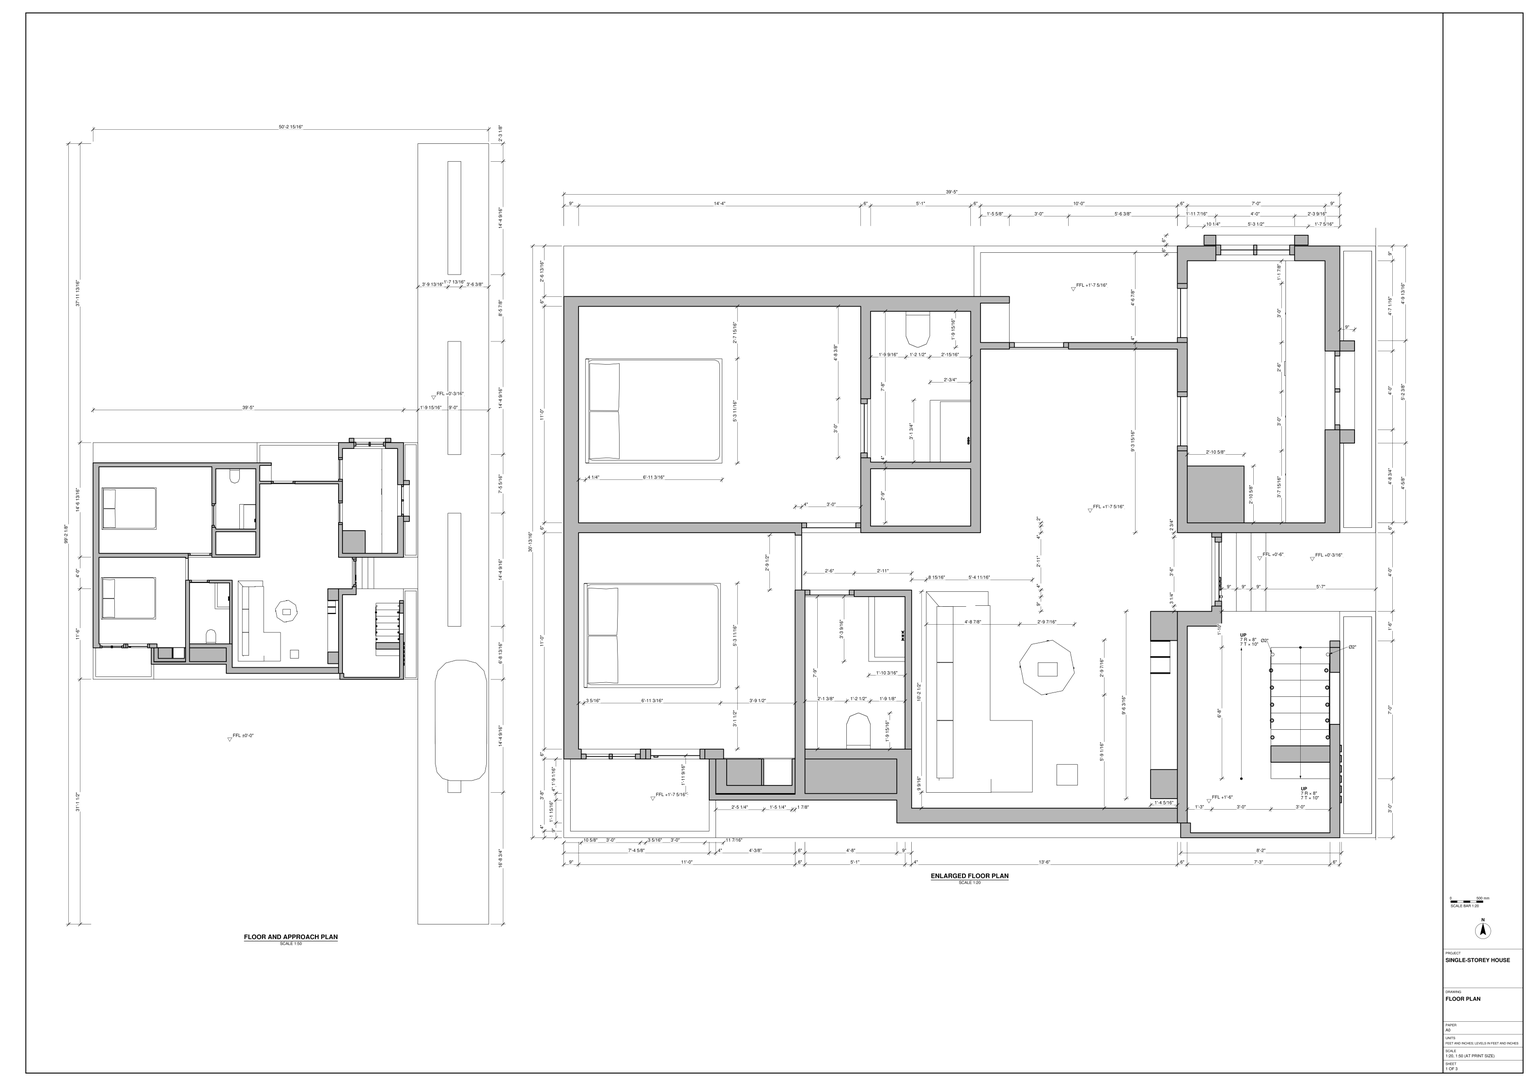
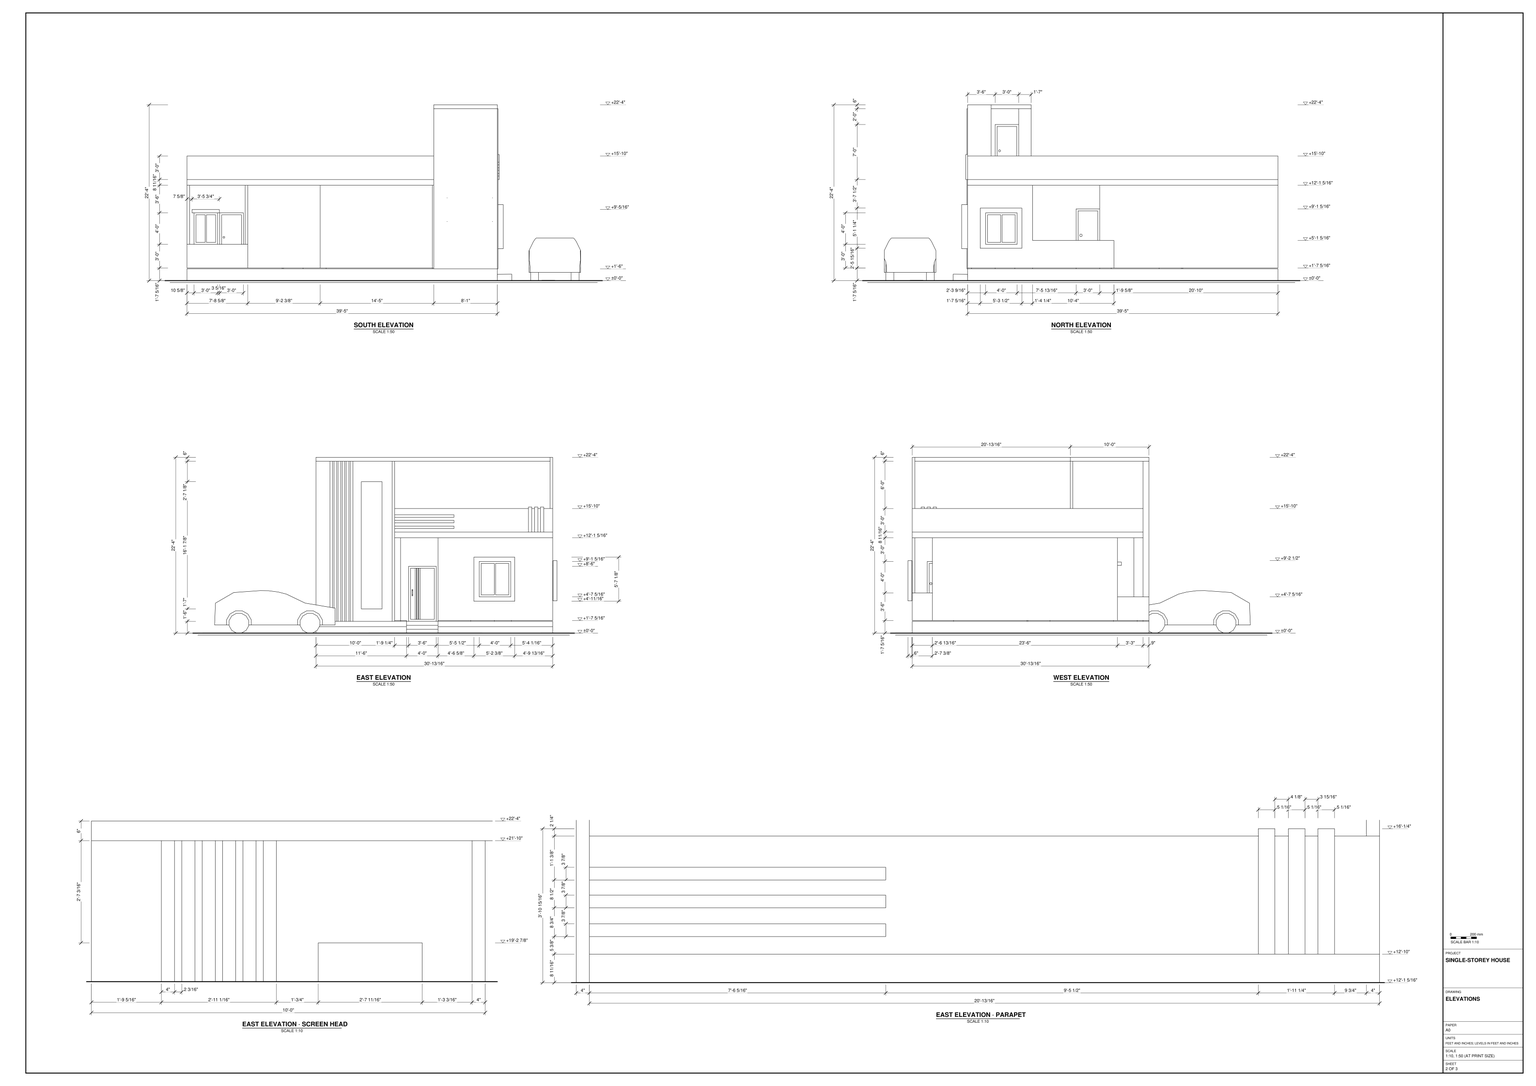
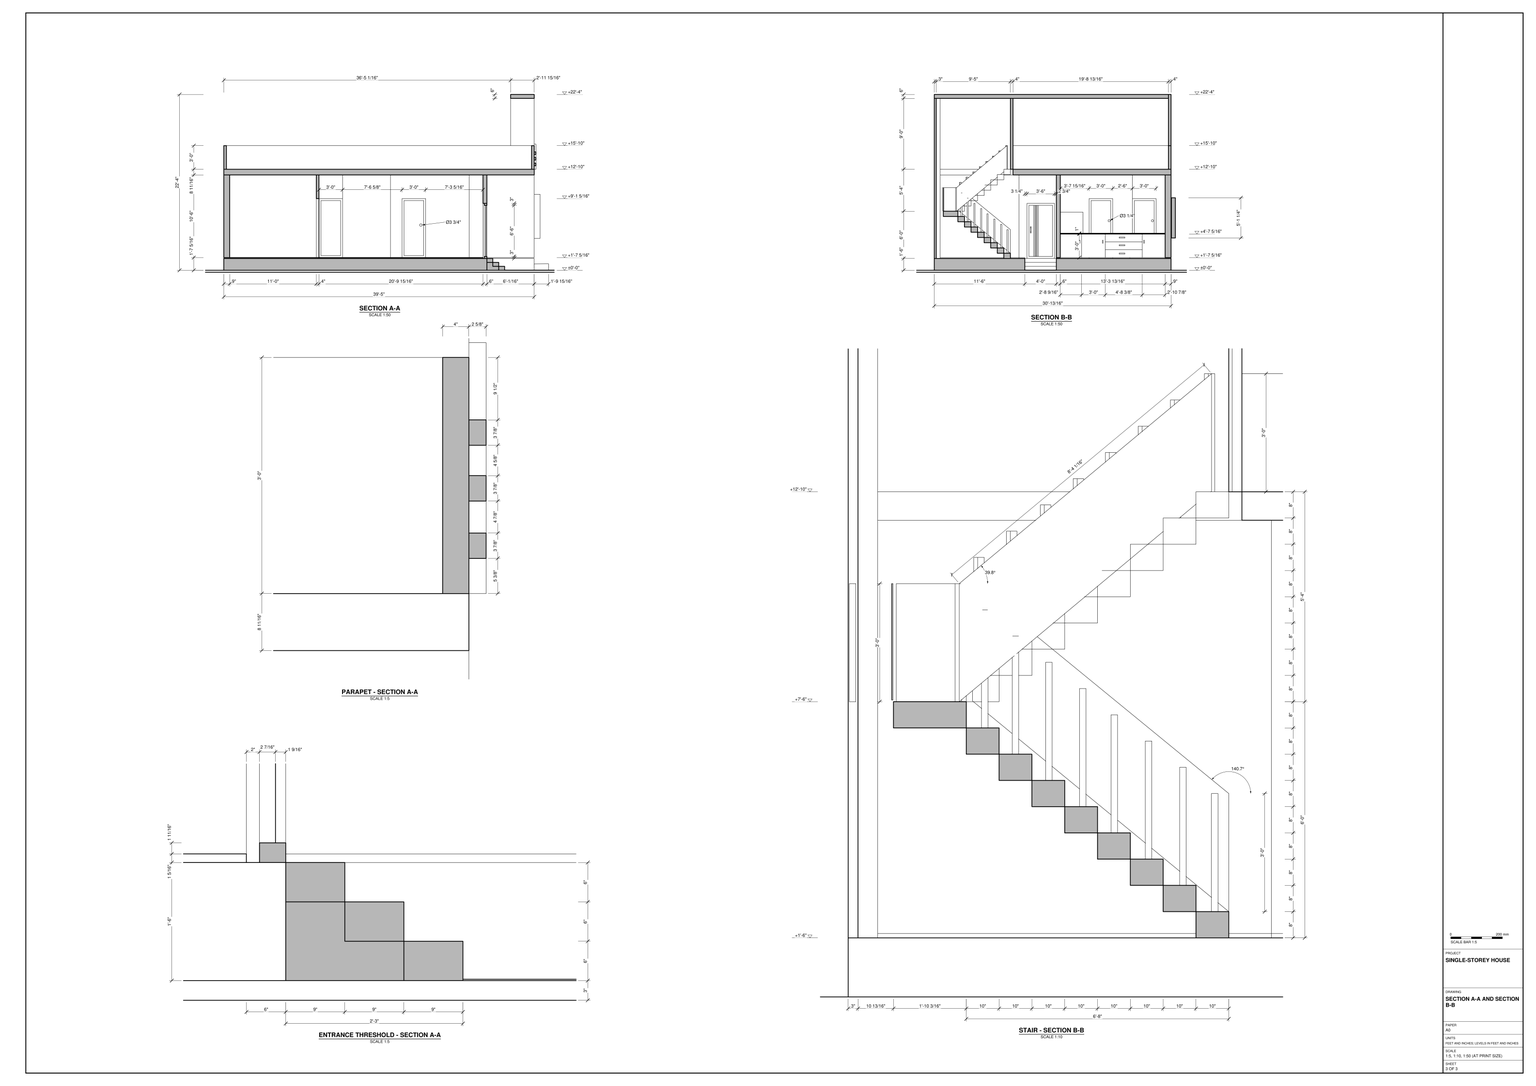
Build the house and its approach in SketchUp using task_files/diagram_01.pdf. Work in feet and inches. The complete model shall measure 379'-4 11/16" along X, 395'-9" along Y and 22'-7" along Z. These are the overall model extents; use the enlarged floor plan to size the house itself. Use ±0'-0" as the single storey reference and follow the sections for the raised floor, entrance steps and roof.

Lay out the two bedrooms on the west side, the adjoining bathroom partitions, the central living area and the rooms and stair bay along the east side. Follow the drawn wall thicknesses and locate the door and window openings from the plan and elevations. Model the floor and roof slabs, parapets and taller stair enclosure. Use the stair section to connect the two flights at the landing and the east elevation details to place the vertical screen and horizontal parapet bands. Include the side approach and the parked car in their plan positions.

Size and place the beds, sectional sofa, low table, shelving and cabinet run to match the drawings, and fit out the bathrooms as shown. Decor and loose items may be represented by any suitable library components. Make the walls, slabs and roof separate groups or components, group each furniture or joinery piece separately, and use components for repeated parts. Save one SketchUp model as output_files/single_storey_house_with_roof_access_and_side_approach.skp.

# SketchUp Ruby script. Lengths in inches.
U = 1.inch
M = Sketchup.active_model
def pt(a) = Geom::Point3d.new(a.map { |v| v * U })
def face(e, loops, mat)
  f = e.add_face(loops[0].map { |a| pt(a) })
  loops[1..].each { |l| e.add_face(l.map { |a| pt(a) }).erase! }
  f.material = f.back_material = mat if mat
  f
end
# faces: each face lists its corners as indices into pts; further lists are holes
def faces(e, pts, list, mat = nil) = list.each { |f| face(e, (f[0].is_a?(Array) ? f : [f]).map { |l| l.map { |i| pts[i] } }, mat) }
# xy, xz, yz: faces in a plane at the given z, y or x. An outline is a flat list of corners, or four numbers for a rectangle; further outlines are holes
def ring(l) = l.size == 4 ? [[l[0], l[1]], [l[2], l[1]], [l[2], l[3]], [l[0], l[3]]] : l.each_slice(2).to_a
def flat(e, list, mat, &to3) = list.each { |f| face(e, (f[0].is_a?(Array) ? f : [f]).map { |l| ring(l).map { |u, v| to3.(u, v) } }, mat) }
def xy(e, z, list, mat = nil) = flat(e, list, mat) { |x, y| [x, y, z] }
def xz(e, y, list, mat = nil) = flat(e, list, mat) { |x, z| [x, y, z] }
def yz(e, x, list, mat = nil) = flat(e, list, mat) { |y, z| [x, y, z] }
def lines(e, pts, list) = list.each { |a, b| e.add_line(pt(pts[a]), pt(pts[b])) }
# prism: a flat outline (further loops are holes) pulled along v
def prism(e, loops, v, mat = nil)
  f = face(e, loops, mat); d = Geom::Vector3d.new(v.map { |x| x * U })
  f.pushpull(f.normal.samedirection?(d) ? d.length : -d.length)
end
def box(e, o, s, mat = nil) = prism(e, [[o, [o[0] + s[0], o[1], o[2]], [o[0] + s[0], o[1] + s[1], o[2]], [o[0], o[1] + s[1], o[2]]]], [0, 0, s[2]], mat)
def at(x, y, z, deg = 0) = Geom::Transformation.translation(pt([x, y, z])) * Geom::Transformation.rotation(ORIGIN, Z_AXIS, deg.degrees)
def axes(o, x, y, z) = Geom::Transformation.new([*x, 0, *y, 0, *z, 0, *pt(o).to_a, 1])
def part(name) = M.definitions.add(name)
# library, detail: a bought-in or finely detailed component or shape, given as its bounding box
def library(name, o, s) = part(name).tap { |d| box(d.entities, o, s) }
def detail(e, o, s) = box(e.add_group.entities, o, s)
def put(e, d, t, mat = nil) = e.add_instance(d, t).tap { |i| i.material = mat if mat }
def group(e, t, mat = nil) = e.add_group.tap { |g| g.transformation = t; g.material = mat if mat }.entities
root = M.entities
M.materials.add("C01_Vanilla_Cream").color = [255, 230, 206]
M.materials.add("D01_Frost_White").color = [255, 242, 206]
M.materials.add("E01_Mint_Frost").color = [255, 255, 204]
M.materials.add("Glass_Basic_01").color = [49, 67, 236]
M.materials["Glass_Basic_01"].alpha = 0.25
M.materials.add("Glass_Basic_1").color = [161, 173, 186]
M.materials["Glass_Basic_1"].alpha = 0.56
M.materials.add("Glass_Sky Reflection_01").color = [126, 138, 183]
M.materials["Glass_Sky Reflection_01"].alpha = 0.25
M.materials.add("M00_Soft_Cloud").color = [255, 255, 255]
M.materials.add("M02_Ash_Whisper").color = [196, 196, 196]
M.materials.add("M03_Pewter_Shine").color = [168, 168, 168]
M.materials.add("M04_Stone_Frost").color = [143, 142, 145]
M.materials.add("M05_Graphite_Haze").color = [114, 114, 114]
M.materials.add("M09_Shadow_Night").color = [0, 0, 0]
M.materials.add("Marble_01_1K").color = [230, 221, 211]
M.materials.add("Marble_03_1K").color = [175, 182, 201]
M.materials.add("Marble_06_1K").color = [165, 150, 147]
M.materials.add("Marble_07_1K").color = [36, 34, 36]
M.materials.add("Marble_20_1K").color = [172, 173, 182]
M.materials.add("Metal_06_1K").color = [238, 236, 231]
M.materials.add("Plywood_01_1K").color = [125, 96, 64]
M.materials.add("Soil_04_1K").color = [152, 146, 88]
M.materials.add("Wood_Floor_01_1K").color = [146, 111, 76]
M.materials.add("Wood_Floor_12_1K").color = [92, 75, 65]
M.materials.add("Wood_Veneer_15_1K").color = [103, 69, 45]
c1 = library("Pouf 005",[-6.34,-6.34,0],[12.68,12.68,13.92])
c2 = library("Table 067",[-16.66,-16.71,0],[33.41,33.42,14.94])
c3 = library("Marcel Lift Bed Queen",[-31.83,-34.39,0],[63.66,83.19,38.98])
c4 = library("Cello Loveseat with Chaise",[-61.38,-32.25,0],[122.52,64.7,30.04])
c5 = library("Railing post",[0,0,0],[2,2,36])
c6 = library("Book 013 Open",[-5.88,-4.14,0],[11.75,8.28,0.91])
c7 = library("Wall Unit 001",[-57.09,-8.46,0],[114.18,16.34,74.8])
c8 = library("Shelf 008",[-36.8125,-5.92,-13.86],[73.625,5.92,27.72])
c9 = library("Toilet 005",[-7.26,-21.97,0],[14.52,21.97,16.93])
c10 = library("Shower Cabin 003",[-0.1,-35.53,0],[35.43,35.43,1.18])
c11 = library("Bathroom Sink 001",[-18.28,-18.5,-10.98],[36.92,18.5,25.55])
c12 = part("Refrigerator 004")
xy(c12.entities,0,[[-17.32,-17.32,-17.32,17.32,17.32,17.32],[-17.32,-17.32,17.32,17.32,17.32,-17.32]])
xy(c12.entities,69.29,[[-17.32,-17.32,17.32,-17.32,17.32,17.32],[-17.32,-17.32,17.32,17.32,-17.32,17.32]])
xz(c12.entities,-17.32,[[-17.32,0,17.32,0,17.32,69.29],[-17.32,0,17.32,69.29,-17.32,69.29]])
xz(c12.entities,17.32,[[-17.32,0,-17.32,69.29,17.32,0],[17.32,0,-17.32,69.29,17.32,69.29]])
yz(c12.entities,-17.32,[[-17.32,0,-17.32,69.29,17.32,0],[17.32,0,-17.32,69.29,17.32,69.29]])
yz(c12.entities,17.32,[[-17.32,0,17.32,0,17.32,69.29],[-17.32,0,17.32,69.29,-17.32,69.29]])
c13 = library("Car 018",[-39.37,-94.12,-0.14],[78.74,183.68,64.54])
c14 = part("Group\#59")
box(c14.entities,[0,0,0],[8.6875,1.6875,0.6875],"Metal_06_1K")
c15 = part("Group\#60")
box(c15.entities,[-0.1875,0,0],[0.1875,1,4.5625],"Metal_06_1K")
c16 = part("Group\#10")
xy(c16.entities,0,[[0,0,36,10]])
c17 = part("Group\#11")
box(c17.entities,[0,0,0],[36,10,8])
c18 = part("Group\#14")
p = [[0,0,100],[0,0,64.23],[0.18,78.12,0],[0.18,78.12,36]]
faces(c18.entities,p,[[0,1,2,3]],"Glass_Basic_01")
c19 = part("Group\#15")
p = [[0,76.9,64.1875],[0,76.9,100],[2.6,0,36],[2.6,0,0]]
faces(c19.entities,p,[[0,1,2,3]])
c20 = library("Group\#16",[-91,0,0],[98,120,244])
c21 = library("Group\#33",[0,-6,0],[36,6,84])
c22 = library("Group\#35",[0,0,0],[4.6,42,84])
c23 = library("Group\#38",[0,0,0],[36,3,90])
c24 = library("Group\#43",[0,0,0],[70.375,3.625,8.5])
c25 = library("Group\#44",[0,0,-4],[162,133,4])
c26 = library("Group\#45",[0,0,-1],[8,8,1])
c27 = library("Group\#46",[0,0,0],[30,3,90])
c28 = library("Group\#47",[-4.77,-0.4375,0],[48.36,23.5625,126])
c29 = library("Group\#58",[-6,0,0],[6,36,90])
c30 = library("Group\#56",[-6,0,0],[6,36,90])
c31 = part("Group\#69")
box(c31.entities,[0,0,0],[2.625,90.3125,3.875])
c32 = part("Group\#73")
box(c32.entities,[0,0,0],[19.8125,172.5625,0.2])
p = [[3264.77,2521.9,90],[3264.77,2521.9,90.23]]
lines(root,p,[[0,1]])
put(root,c1,at(3105.04,2526.62,19.3125))
put(root,c2,at(3092.74,2592.07,19.3125))
put(root,c3,at(2859.35,2611.64,19.3125,90))
put(root,c3,at(2860.3125,2748.52,19.3125,90))
put(root,c4,at(3051.63,2577.23,19.3125,90))
put(root,c5,at(3262.95,2599.03,26))
put(root,c5,at(3262.04,2589.34,34))
put(root,c5,at(3262.55,2578.86,42))
put(root,c5,at(3262.67,2568.42,50))
put(root,c5,at(3262.6,2558.81,58))
put(root,c5,at(3262.88,2548.48,66))
put(root,c5,at(3262.58,2538.29,74))
put(root,c5,at(3262.63,2528.94,82))
put(root,c5,at(3262.77,2520.9,90))
put(root,c5,at(3262.77,2488.65,90))
put(root,c5,at(3193.65,2488.65,90))
put(root,c5,at(3226.38,2527.78,98))
put(root,c5,at(3226.14,2537.75,106))
put(root,c5,at(3226.8,2548.08,114))
put(root,c5,at(3226.53,2558.08,122))
put(root,c5,at(3226.55,2567.91,130))
put(root,c5,at(3226.55,2577.91,138))
put(root,c5,at(3226.51,2587.72,146))
put(root,c5,at(3226.4375,2598.0625,154))
put(root,c5,at(3194.21,2596.86,154))
put(root,c5,at(3194.32,2576.72,138))
put(root,c5,at(3194.32,2566.72,130))
put(root,c5,at(3194.15,2526.58,98))
put(root,c5,at(3194.31,2556.89,122))
put(root,c5,at(3194.58,2546.89,114))
put(root,c5,at(3193.91,2536.56,106))
put(root,c5,at(3194.28,2586.52,146))
put(root,c5,at(3229.25,2599.03,26))
put(root,c5,at(3228.34,2589.34,34))
put(root,c5,at(3229.07,2520.9,90))
put(root,c5,at(3228.85,2578.86,42))
put(root,c5,at(3229.18,2548.48,66))
put(root,c5,at(3228.9,2558.81,58))
put(root,c5,at(3228.97,2568.42,50))
put(root,c5,at(3228.88,2538.29,74))
put(root,c5,at(3228.93,2528.94,82))
put(root,c6,at(3093.23,2590.97,33.09))
put(root,c7,at(3163.79,2569.23,35.9375,90))
put(root,c8,at(3088.99,2512.23,94.84))
put(root,c9,at(2977.88,2542.3125,20.49,180))
put(root,c10,axes([2945.42,2635.57,19.3125],[1.72156,0,0],[0,2.62467,0],[0,0,1]))
put(root,c11,at(3006.25,2617.03,57.48,-90))
put(root,c10,axes([2985.42,2810.57,19.3125],[1.72156,0,0],[0,2.62467,0],[0,0,1]))
put(root,c9,at(3014.05,2809.3125,24.35))
put(root,c11,at(3046.25,2735.95,58.17,-90))
put(root,c12,at(3195.57,2697.64,19.3125,-180))
put(root,c13,at(3358.8,2427.97,0.4))
g1 = group(root,at(2798.25,2488.3125,19.3125),"C01_Vanilla_Cream")
g2 = group(g1,at(0,0,-1.3125),"C01_Vanilla_Cream")
xy(g2,0,[[374,9,380,129],[212,18,374,18,374,138,400.9375,138,400.9375,141.25,394.9375,141.25,394.9375,183.25,400.9375,183.25,400.9375,186,374,186,374,297.9375,254,297.9375,254,186,145,186,145,151,212,151]])
xy(g2,1.3125,[[4,4,88.64,4,88.64,48,85.95,48,85.95,54,49.95,54,49.95,48,4,48],[203,9,374,18],[374,9,380,129],[[212,18,374,18,374,138,394.9375,138,394.9375,186,473,186,473,360.8125,250,360.8125,250,330,0,330,0,48,46.64,48,46.64,54,9,54,9,186,141,186,141,184.48,145,184.48,145,151,177,151,177,147,208,147,208,54,212,54],[380,192,380,235.91,374,235.91,374,271.91,380,271.91,380,301.9375,307.625,301.9375,307.625,297.9375,271.625,297.9375,271.625,301.9375,254,301.9375,254,326,271.625,326,271.625,330,254,330,254,356.8125,374,356.8125,374,337.9375,380,337.9375,380,351.8125,464,351.8125,464,192],[187,229,187,231.65,181,231.65,181,267.65,187,267.65,187,321,248,321,248,229],[187,190,248,225],[145,186,181,192]],[141,22.9375,147,151],
  [92.64,26.9375,141,26.9375,141,186,9,186,9,54,97.41,54,97.41,48,92.64,48],[147,26.9375,203,48],[88.64,48,97.41,54],[147,54,208,147],[147,147,177,151],
  [141,151,145,184.48],[145,186,181,192],[187,190,248,225],[9,192,181,324],[380,192,440,351.8125],
  [187,229,248,321],[181,231.65,187,267.65],[374,235.91,380,271.91],[271.625,297.9375,307.625,301.9375],[254,301.9375,271.625,326],
  [271.625,301.9375,374,301.9375,374,356.8125,254,356.8125,254,330,271.625,330],[374,301.9375,380,337.9375]])
xy(g2,1.3125,[[92.64,22.9375,141,26.9375]],"E01_Mint_Frost")
xy(g2,37.3125,[[0,0,92.64,0,92.64,22.9375,88.64,22.9375,88.64,4,4,4,4,48,0,48]])
xy(g2,37.3125,[[10.64,48,46.64,54],[464,248.75,473,296.75],[397.4375,351.8125,445.4375,360.8125]],"D01_Frost_White")
xy(g2,37.3125,[[440,192,464,351.8125]],"Marble_07_1K")
xy(g2,38.3125,[[440,192,464,351.8125]],"Marble_07_1K")
xy(g2,43.3125,[[250,330,254,330,254,356.8125,374,356.8125,374,360.8125,250,360.8125]],"D01_Frost_White")
xy(g2,84,[[394.9375,141.25,400.9375,183.25]],"D01_Frost_White")
xy(g2,85.3125,[[10.64,48,46.64,54],[49.95,48,85.95,54],[172.37,48,197.74,54],[397.4375,351.8125,445.4375,360.8125]],"D01_Frost_White")
xy(g2,91.3125,[[147,147,177,151],[141,151,145,184.48],[145,186,181,192],[181,231.65,187,267.65],[374,235.91,380,271.91],
  [464,248.75,473,296.75],[271.625,297.9375,307.625,301.9375],[374,301.9375,380,337.9375]],"D01_Frost_White")
xy(g2,109.3125,[[172.37,48,197.74,54]],"D01_Frost_White")
xy(g2,127.3125,[[203,9,374,9,374,18,212,18,212,54,147,54,147,48,203,48],[374,9,380,129],[88.64,22.9375,92.64,48],[92.64,22.9375,203,22.9375,203,26.9375,147,26.9375,147,151,141,151,141,26.9375,92.64,26.9375],[[0,48,97.41,48,97.41,54,9,54,9,186,141,186,141,151,145,151,145,186,254,186,254,297.9375,374,297.9375,374,186,473,186,473,360.8125,374,360.8125,374,301.9375,380,301.9375,380,351.8125,464,351.8125,464,192,380,192,380,301.9375,254,301.9375,254,326,271.625,326,271.625,330,0,330],[9,192,181,324],[187,229,248,321],[187,190,248,225]],
  [208,54,212,54,212,151,147,151,147,147,208,147],[374,129,400.9375,138],[394.9375,138,400.9375,186]],"D01_Frost_White")
xz(g2,0,[[0,1.3125,92.64,37.3125]])
xz(g2,4,[[4,1.3125,88.64,37.3125]])
xz(g2,9,[[203,1.3125,374,127.3125]],"C01_Vanilla_Cream")
xz(g2,9,[[374,0,380,127.3125]],"D01_Frost_White")
xz(g2,18,[[212,0,374,1.3125]])
xz(g2,18,[[212,1.3125,374,127.3125]],"D01_Frost_White")
xz(g2,22.9375,[[92.64,1.3125,203,127.3125],[88.64,37.3125,92.64,127.3125]],"C01_Vanilla_Cream")
xz(g2,26.9375,[[92.64,1.3125,141,127.3125],[147,1.3125,203,127.3125]],"D01_Frost_White")
xz(g2,48,[[0,1.3125,4,37.3125]])
xz(g2,48,[[[4,1.3125,49.95,1.3125,49.95,85.3125,85.95,85.3125,85.95,1.3125,88.64,1.3125,88.64,127.3125,4,127.3125],[10.64,37.3125,46.64,85.3125]],[0,37.3125,4,127.3125]],"C01_Vanilla_Cream")
xz(g2,48,[[92.64,1.3125,97.41,127.3125],[[147,1.3125,203,127.3125],[172.37,85.3125,197.74,109.3125]]],"D01_Frost_White")
xz(g2,48,[[88.64,1.3125,92.64,127.3125]],"E01_Mint_Frost")
xz(g2,54,[[[9,1.3125,9,127.3125,97.41,127.3125,97.41,1.3125,85.95,1.3125,85.95,85.3125,49.95,85.3125,49.95,1.3125],[10.64,37.3125,46.64,85.3125]],[[147,1.3125,208,127.3125],[172.37,85.3125,197.74,109.3125]]],"D01_Frost_White")
xz(g2,54,[[208,1.3125,212,127.3125]],"E01_Mint_Frost")
xz(g2,129,[[374,0,380,1.3125]])
xz(g2,129,[[380,1.3125,400.9375,127.3125]],"C01_Vanilla_Cream")
xz(g2,138,[[374,1.3125,394.9375,127.3125]],"D01_Frost_White")
xz(g2,141.25,[[394.9375,0,400.9375,84]],"D01_Frost_White")
xz(g2,147,[[177,1.3125,208,1.3125,208,127.3125,147,127.3125,147,91.3125,177,91.3125]],"D01_Frost_White")
xz(g2,151,[[145,0,147,1.3125],[147,0,177,1.3125]])
xz(g2,151,[[177,0,177,91.3125,147,91.3125,147,127.3125,212,127.3125,212,0],[141,1.3125,145,91.3125],[145,1.3125,147,127.3125]],"D01_Frost_White")
xz(g2,183.25,[[394.9375,0,400.9375,84]],"D01_Frost_White")
xz(g2,184.48,[[141,1.3125,145,91.3125]],"D01_Frost_White")
xz(g2,186,[[145,0,147,1.3125],[147,0,181,1.3125],[394.9375,1.3125,400.9375,127.3125]])
xz(g2,186,[[400.9375,1.3125,473,127.3125]],"C01_Vanilla_Cream")
xz(g2,186,[[181,0,254,127.3125],[374,0,400.9375,0,400.9375,1.3125,394.9375,1.3125,394.9375,127.3125,374,127.3125],[9,1.3125,141,127.3125],[145,91.3125,181,127.3125]],"D01_Frost_White")
xz(g2,190,[[187,1.3125,248,127.3125]],"D01_Frost_White")
xz(g2,192,[[440,1.3125,464,37.3125]])
xz(g2,192,[[9,1.3125,9,127.3125,181,127.3125,181,91.3125,145,91.3125,145,1.3125],[380,1.3125,380,127.3125,464,127.3125,464,38.3125,440,38.3125,440,1.3125]],"D01_Frost_White")
xz(g2,192,[[440,37.3125,464,38.3125]],"Marble_07_1K")
xz(g2,225,[[187,1.3125,248,127.3125]],"D01_Frost_White")
xz(g2,229,[[187,1.3125,248,127.3125]],"D01_Frost_White")
xz(g2,231.65,[[181,1.3125,187,91.3125]],"D01_Frost_White")
xz(g2,235.91,[[374,1.3125,380,91.3125]],"D01_Frost_White")
xz(g2,248.75,[[464,37.3125,473,91.3125]],"D01_Frost_White")
xz(g2,267.65,[[181,1.3125,187,91.3125]],"D01_Frost_White")
xz(g2,271.91,[[374,1.3125,380,91.3125]],"D01_Frost_White")
xz(g2,296.75,[[464,37.3125,473,91.3125]],"D01_Frost_White")
xz(g2,297.9375,[[271.625,0,307.625,1.3125]])
xz(g2,297.9375,[[254,0,271.625,0,271.625,91.3125,307.625,91.3125,307.625,0,374,0,374,127.3125,254,127.3125]],"D01_Frost_White")
xz(g2,301.9375,[[254,1.3125,254,127.3125,374,127.3125,374,1.3125,307.625,1.3125,307.625,91.3125,271.625,91.3125,271.625,1.3125]],"C01_Vanilla_Cream")
xz(g2,301.9375,[[374,1.3125,380,91.3125]],"D01_Frost_White")
xz(g2,321,[[187,1.3125,248,127.3125]],"D01_Frost_White")
xz(g2,324,[[9,1.3125,181,127.3125]],"D01_Frost_White")
xz(g2,326,[[254,1.3125,271.625,127.3125]],"D01_Frost_White")
xz(g2,330,[[0,1.3125,0,127.3125,271.625,127.3125,271.625,1.3125,254,1.3125,254,43.3125,250,43.3125,250,1.3125]],"C01_Vanilla_Cream")
xz(g2,337.9375,[[374,1.3125,380,91.3125]],"D01_Frost_White")
xz(g2,351.8125,[[440,1.3125,464,37.3125]])
xz(g2,351.8125,[[380,1.3125,440,1.3125,440,37.3125,397.4375,37.3125,397.4375,85.3125,445.4375,85.3125,445.4375,38.3125,464,38.3125,464,127.3125,380,127.3125]],"D01_Frost_White")
xz(g2,351.8125,[[440,37.3125,445.4375,38.3125],[445.4375,37.3125,464,38.3125]],"Marble_07_1K")
xz(g2,356.8125,[[254,1.3125,374,43.3125]],"D01_Frost_White")
xz(g2,360.8125,[[[250,1.3125,250,43.3125,374,43.3125,374,127.3125,473,127.3125,473,1.3125],[397.4375,37.3125,445.4375,85.3125]]],"C01_Vanilla_Cream")
yz(g2,0,[[0,1.3125,48,37.3125]])
yz(g2,0,[[48,1.3125,330,127.3125]],"C01_Vanilla_Cream")
yz(g2,4,[[4,1.3125,48,37.3125]])
yz(g2,9,[[54,1.3125,186,127.3125],[192,1.3125,324,127.3125]],"D01_Frost_White")
yz(g2,10.64,[[48,37.3125,54,85.3125]],"D01_Frost_White")
yz(g2,46.64,[[48,37.3125,54,85.3125]],"D01_Frost_White")
yz(g2,49.95,[[48,1.3125,54,85.3125]],"D01_Frost_White")
yz(g2,85.95,[[48,1.3125,54,85.3125]],"D01_Frost_White")
yz(g2,88.64,[[4,1.3125,22.9375,37.3125]])
yz(g2,88.64,[[22.9375,1.3125,48,127.3125]],"C01_Vanilla_Cream")
yz(g2,92.64,[[0,1.3125,22.9375,37.3125]])
yz(g2,92.64,[[26.9375,1.3125,48,127.3125]],"D01_Frost_White")
yz(g2,97.41,[[48,1.3125,54,127.3125]],"D01_Frost_White")
yz(g2,141,[[26.9375,1.3125,151,127.3125],[184.48,1.3125,184.48,91.3125,151,91.3125,151,127.3125,186,127.3125,186,1.3125]],"D01_Frost_White")
yz(g2,145,[[151,0,184.48,1.3125]])
yz(g2,145,[[184.48,0,186,0,186,127.3125,151,127.3125,151,91.3125,184.48,91.3125],[186,1.3125,192,91.3125]],"D01_Frost_White")
yz(g2,147,[[26.9375,1.3125,48,127.3125],[54,1.3125,147,127.3125],[147,1.3125,151,91.3125]],"D01_Frost_White")
yz(g2,147,[[48,1.3125,54,127.3125]],"E01_Mint_Frost")
yz(g2,172.37,[[48,85.3125,54,109.3125]],"D01_Frost_White")
yz(g2,177,[[147,1.3125,151,91.3125]],"D01_Frost_White")
yz(g2,181,[[186,1.3125,192,91.3125],[192,1.3125,192,127.3125,324,127.3125,324,1.3125,267.65,1.3125,267.65,91.3125,231.65,91.3125,231.65,1.3125]],"D01_Frost_White")
yz(g2,187,[[190,1.3125,225,127.3125],[229,1.3125,231.65,1.3125,231.65,91.3125,267.65,91.3125,267.65,1.3125,321,1.3125,321,127.3125,229,127.3125]],"D01_Frost_White")
yz(g2,197.74,[[48,85.3125,54,109.3125]],"D01_Frost_White")
yz(g2,203,[[9,1.3125,22.9375,127.3125]],"C01_Vanilla_Cream")
yz(g2,203,[[26.9375,1.3125,48,127.3125]],"D01_Frost_White")
yz(g2,208,[[54,1.3125,147,127.3125]],"D01_Frost_White")
yz(g2,212,[[18,0,54,1.3125]])
yz(g2,212,[[54,0,151,127.3125],[18,1.3125,54,127.3125]],"D01_Frost_White")
yz(g2,248,[[190,1.3125,225,127.3125],[229,1.3125,321,127.3125]],"D01_Frost_White")
yz(g2,250,[[330,1.3125,360.8125,43.3125]],"C01_Vanilla_Cream")
yz(g2,254,[[301.9375,1.3125,326,127.3125]],"C01_Vanilla_Cream")
yz(g2,254,[[186,0,297.9375,127.3125],[330,1.3125,356.8125,43.3125]],"D01_Frost_White")
yz(g2,271.625,[[297.9375,1.3125,301.9375,91.3125],[326,1.3125,330,127.3125]],"D01_Frost_White")
yz(g2,307.625,[[297.9375,1.3125,301.9375,91.3125]],"E01_Mint_Frost")
yz(g2,374,[[9,0,18,1.3125],[18,0,129,1.3125],[129,0,138,1.3125],[235.91,0,271.91,1.3125]])
yz(g2,374,[[337.9375,1.3125,337.9375,91.3125,301.9375,91.3125,301.9375,127.3125,356.8125,127.3125,356.8125,1.3125],[356.8125,43.3125,360.8125,127.3125]],"C01_Vanilla_Cream")
yz(g2,374,[[186,0,186,127.3125,297.9375,127.3125,297.9375,0,271.91,0,271.91,91.3125,235.91,91.3125,235.91,0],[18,1.3125,138,127.3125]],"D01_Frost_White")
yz(g2,374,[[9,1.3125,18,127.3125]],"E01_Mint_Frost")
yz(g2,380,[[9,0,129,127.3125]],"C01_Vanilla_Cream")
yz(g2,380,[[192,1.3125,235.91,1.3125,235.91,91.3125,271.91,91.3125,271.91,1.3125,301.9375,1.3125,301.9375,127.3125,192,127.3125],[337.9375,1.3125,351.8125,1.3125,351.8125,127.3125,301.9375,127.3125,301.9375,91.3125,337.9375,91.3125]],"D01_Frost_White")
yz(g2,394.9375,[[141.25,0,183.25,1.3125],[138,1.3125,138,127.3125,186,127.3125,186,1.3125,183.25,1.3125,183.25,84,141.25,84,141.25,1.3125]],"D01_Frost_White")
yz(g2,397.4375,[[351.8125,37.3125,360.8125,85.3125]],"D01_Frost_White")
yz(g2,400.9375,[[138,0,138,1.3125,129,1.3125,129,127.3125,186,127.3125,186,0,183.25,0,183.25,84,141.25,84,141.25,0]],"D01_Frost_White")
yz(g2,440,[[192,1.3125,224.5625,37.3125],[224.5625,1.3125,260.5625,37.3125],[260.5625,1.3125,316.9375,13.3125],[316.9375,1.3125,351.8125,37.3125],[260.5625,13.3125,316.9375,25.3125],
  [260.5625,25.3125,316.9375,37.3125]])
yz(g2,440,[[192,37.3125,351.8125,38.3125]],"Marble_07_1K")
yz(g2,445.4375,[[351.8125,37.3125,360.8125,85.3125]],"D01_Frost_White")
yz(g2,464,[[192,1.3125,351.8125,37.3125]])
yz(g2,464,[[192,38.3125,192,127.3125,351.8125,127.3125,351.8125,38.3125,296.75,38.3125,296.75,91.3125,248.75,91.3125,248.75,38.3125]],"D01_Frost_White")
yz(g2,464,[[192,37.3125,248.75,38.3125],[248.75,37.3125,296.75,38.3125],[296.75,37.3125,351.8125,38.3125]],"Marble_07_1K")
yz(g2,473,[[[186,1.3125,360.8125,127.3125],[248.75,37.3125,296.75,91.3125]]],"C01_Vanilla_Cream")
p = [[145,192,91.3125],[145,192.1875,91.3125]]
lines(g2,p,[[0,1]])
put(g2,c14,axes([440,290.43,31.02],[0,-1,0],[0,0,1],[-1,0,0]))
put(g2,c14,axes([440,290.43,19.27],[0,-1,0],[0,0,1],[-1,0,0]))
put(g2,c14,axes([440,290.43,6.65],[0,-1,0],[0,0,1],[-1,0,0]))
put(g1,c15,at(440,319.11,21.96))
put(g1,c15,at(440,256.3,21.96))
put(g1,c15,at(440,220.98,21.96))
g3 = group(root,at(2321.5625,2217.6875,0),"Marble_20_1K")
xy(g3,-3,[[-2321.5625,-2217.6875,2231.125,2531.3125]])
xy(g3,0,[[476.6875,270.625,949.6875,270.625,949.6875,408.625,877.625,408.625,877.625,456.625,949.6875,456.625,949.6875,631.4375,476.6875,631.4375]])
xy(g3,0,[[[-2321.5625,-2217.6875,2231.125,2531.3125],[476.6875,270.625,476.6875,631.4375,949.6875,631.4375,949.6875,456.625,877.625,456.625,877.625,408.625,949.6875,408.625,949.6875,270.625]]],"Soil_04_1K")
xy(g3,18,[[476.6875,270.625,949.6875,270.625,949.6875,408.625,877.625,408.625,877.625,456.625,949.6875,456.625,949.6875,631.4375,476.6875,631.4375]],"M03_Pewter_Shine")
xz(g3,-2217.6875,[[-2321.5625,-3,2231.125,0]])
xz(g3,270.625,[[476.6875,0,949.6875,18]],"M03_Pewter_Shine")
xz(g3,408.625,[[877.625,0,949.6875,18]],"M03_Pewter_Shine")
xz(g3,456.625,[[877.625,0,949.6875,18]],"M03_Pewter_Shine")
xz(g3,631.4375,[[476.6875,0,949.6875,18]],"M03_Pewter_Shine")
xz(g3,2531.3125,[[-2321.5625,-3,2231.125,0]])
yz(g3,-2321.5625,[[-2217.6875,-3,2531.3125,0]])
yz(g3,476.6875,[[270.625,0,631.4375,18]],"M03_Pewter_Shine")
yz(g3,877.625,[[408.625,0,456.625,18]])
yz(g3,949.6875,[[270.625,0,408.625,18],[456.625,0,631.4375,18]],"M03_Pewter_Shine")
yz(g3,2231.125,[[-2217.6875,-3,2531.3125,0]])
g4 = group(root,at(3199.1875,2629.5625,18),"Marble_06_1K")
box(g4,[0,-3.25,-6],[9,48,6])
g5 = group(root,at(3208.1875,2629.5625,12),"Marble_06_1K")
box(g5,[0,-3.25,-6],[9,48,6])
g6 = group(root,at(3217.1875,2629.5625,6),"Marble_06_1K")
box(g6,[0,-3.25,-6],[9,48,6])
g7 = group(root,at(3229.25,2524.3125,18))
xy(g7,0,[[0,0,36,10]])
put(root,c16,at(3229.25,2534.3125,18))
put(root,c16,at(3229.25,2544.3125,18))
put(root,c16,at(3229.25,2574.3125,18))
put(root,c16,at(3229.25,2584.3125,18))
put(root,c17,at(3229.25,2594.3125,18))
put(root,c17,at(3229.25,2584.3125,26))
put(root,c17,at(3229.25,2574.3125,34))
put(root,c17,at(3229.25,2564.3125,42))
put(root,c17,at(3229.25,2554.3125,50))
put(root,c17,at(3229.25,2544.3125,58))
put(root,c17,at(3229.25,2534.3125,66))
put(root,c17,at(3229.25,2524.3125,74))
g8 = group(root,at(3229.25,2514.3125,82))
box(g8,[-36,-12.1875,0],[72,22.1875,8])
put(root,c17,at(3193.25,2524.3125,90))
put(root,c17,at(3193.25,2534.3125,98))
put(root,c17,at(3193.25,2544.3125,106))
put(root,c17,at(3193.25,2554.3125,114))
put(root,c17,at(3193.25,2564.3125,122))
put(root,c17,at(3193.25,2574.3125,130))
put(root,c17,at(3193.25,2584.3125,138))
put(root,c17,at(3193.25,2594.3125,146))
g9 = group(root,at(2798.25,2536.3125,145.3125),"C01_Vanilla_Cream")
xy(g9,0,[[0,-39,0,312.8125,473,312.8125,473,72,380,72,380,-39]])
xy(g9,8.6875,[[0,-39,0,312.8125,473,312.8125,473,72,469,72,469,308.8125,4,308.8125,4,-35,376,-35,376,-39],[376,-39,380,68],[4,-35,376,-35,376,72,469,72,469,308.8125,4,308.8125],[376,68,380,72],[380,68,395,72]])
xy(g9,44.6875,[[0,-39,376,-39,376,-35,4,-35,4,308.8125,469,308.8125,469,72,473,72,473,312.8125,0,312.8125]])
xy(g9,116.6875,[[376,-39,380,68],[376,68,395,72]])
xz(g9,-39,[[376,8.6875,380,116.6875]])
xz(g9,-39,[[0,8.6875,376,44.6875]],"M02_Ash_Whisper")
xz(g9,-39,[[0,0,380,8.6875]],"M03_Pewter_Shine")
xz(g9,-35,[[4,8.6875,376,44.6875]])
xz(g9,68,[[376,8.6875,380,116.6875],[380,8.6875,395,116.6875]])
xz(g9,72,[[380,0,473,8.6875],[376,8.6875,395,116.6875],[469,8.6875,473,44.6875]])
xz(g9,308.8125,[[4,8.6875,469,44.6875]])
xz(g9,312.8125,[[0,8.6875,473,44.6875]],"M02_Ash_Whisper")
xz(g9,312.8125,[[0,0,473,8.6875]],"M03_Pewter_Shine")
yz(g9,0,[[-39,8.6875,312.8125,44.6875]],"M02_Ash_Whisper")
yz(g9,0,[[-39,0,312.8125,8.6875]],"M03_Pewter_Shine")
yz(g9,4,[[-35,8.6875,308.8125,44.6875]])
yz(g9,376,[[-35,8.6875,-35,44.6875,-39,44.6875,-39,116.6875,68,116.6875,68,8.6875],[-39,8.6875,-35,44.6875],[68,8.6875,72,116.6875]])
yz(g9,380,[[-39,0,72,8.6875],[-39,8.6875,68,116.6875]])
yz(g9,395,[[68,8.6875,72,116.6875]])
yz(g9,469,[[72,8.6875,308.8125,44.6875]])
yz(g9,473,[[72,8.6875,294.03,44.6875],[299.1,8.6875,312.8125,44.6875]],"M02_Ash_Whisper")
yz(g9,473,[[72,0,312.8125,8.6875]],"M03_Pewter_Shine")
g10 = group(g9,at(473,294.03,8.6875))
box(g10,[0,0,0],[2.625,5.07,38.25],"M00_Soft_Cloud")
g11 = group(g9,at(473,285.03,8.6875))
box(g11,[0,0,0],[2.625,5.07,38.25],"M00_Soft_Cloud")
g12 = group(g9,at(473,275.84,8.6875))
box(g12,[0,0,0],[2.625,5.07,38.25],"M00_Soft_Cloud")
g13 = group(root,at(3193.25,2501.5,90),"Glass_Basic_01")
p = [[2.4,33.53,36],[2.4,1.47,36],[0,1.47,0],[0,33.53,0],[71.52,1.47,36],[71.52,1.47,0],
  [71.39,33.22,0],[71.39,33.22,36],[71.48,0,36],[1.14,0.5,36],[1.14,0.5,0.51],[71.48,0,0.51]]
faces(g13,p,[[0,1,2,3],[4,5,6,7],[8,9,10,11]])
put(root,c16,at(3229.25,2554.3125,18))
put(root,c16,at(3229.25,2564.3125,18))
put(root,c18,at(3264.77,2521.9,26))
put(root,c18,at(3229.07,2526.19,26))
put(root,c19,at(3228.4375,2522.16,90),"Glass_Basic_01")
put(root,c19,at(3190.65,2522.16,90),"Glass_Basic_01")
put(root,c20,at(3265.25,2488.3125,18),"D01_Frost_White")
g14 = group(root,at(3174.25,2488.3125,262),"M05_Graphite_Haze")
xy(g14,-72,[[61.0625,356.8125,97,360.8125]])
xy(g14,0,[[0,0,0,120,61.0625,120,61.0625,356.8125,97,356.8125,97,0]])
xy(g14,6,[[0,0,97,0,97,356.8125,61.0625,356.8125,61.0625,120,0,120],[61.0625,356.8125,97,360.8125]])
xz(g14,0,[[0,0,97,6]])
xz(g14,120,[[0,0,61.0625,6]])
xz(g14,356.8125,[[61.0625,-72,97,0],[61.0625,0,97,6]])
xz(g14,360.8125,[[61.0625,-72,97,6]])
yz(g14,0,[[0,0,120,6]])
yz(g14,61.0625,[[356.8125,-72,360.8125,6],[120,0,356.8125,6]])
yz(g14,97,[[356.8125,-72,360.8125,6],[0,0,356.8125,6]])
g15 = group(root,at(3271.25,2557.4375,36.97))
yz(g15,0,[[0,0,31.6875,193.875]],"Glass_Basic_01")
g16 = group(root,at(3268.25,2737.0625,55.3125))
xy(g16,0,[[0,0,3,48]],"Wood_Floor_12_1K")
xy(g16,3,[[0,3,3,23],[0,25,3,45]],"Wood_Floor_12_1K")
xy(g16,51,[[0,3,3,23],[0,25,3,45]],"Wood_Floor_12_1K")
xy(g16,54,[[0,0,3,48]],"Wood_Floor_12_1K")
xz(g16,0,[[0,0,3,54]],"Wood_Floor_12_1K")
xz(g16,3,[[0,3,3,51]],"Wood_Floor_12_1K")
xz(g16,23,[[0,3,3,51]],"Wood_Floor_12_1K")
xz(g16,25,[[0,3,3,51]],"Wood_Floor_12_1K")
xz(g16,45,[[0,3,3,51]],"Wood_Floor_12_1K")
xz(g16,48,[[0,0,3,54]],"Wood_Floor_12_1K")
yz(g16,0,[[3,3,23,51],[25,3,45,51]],"Glass_Sky Reflection_01")
yz(g16,0,[[[0,0,48,54],[3,3,23,51],[25,3,45,51]]],"Wood_Floor_12_1K")
yz(g16,3,[[[0,0,48,54],[3,3,23,51],[25,3,45,51]]],"Wood_Floor_12_1K")
g17 = group(root,at(3271.25,2737.0625,55.3125))
prism(g17,[[[0,-8.14,60.48],[0,54.24,60.48],[0,54.24,-6.65],[0,-8.14,-6.65]],[[0,48,54],[0,0,54],[0,0,0],[0,48,0]]],[9,0,0],"M04_Stone_Frost")
g18 = group(root,at(3195.6875,2843.6875,55.3125))
xy(g18,0,[[0,0,48,6]],"Wood_Floor_12_1K")
xy(g18,3,[[3,0,23,3],[25,0,45,3],[3,3,23,6],[25,3,45,6]],"Wood_Floor_12_1K")
xy(g18,45,[[3,0,23,3],[25,0,45,3],[3,3,23,6],[25,3,45,6]],"Wood_Floor_12_1K")
xy(g18,48,[[0,0,48,6]],"Wood_Floor_12_1K")
xz(g18,0,[[[0,0,48,48],[25,3,45,45],[3,3,23,45]]],"Wood_Floor_12_1K")
xz(g18,3,[[3,3,45,45]],"Glass_Sky Reflection_01")
xz(g18,6,[[[0,0,48,48],[25,3,45,45],[3,3,23,45]]],"Wood_Floor_12_1K")
yz(g18,0,[[0,0,6,48]],"Wood_Floor_12_1K")
yz(g18,3,[[0,3,3,45],[3,3,6,45]],"Wood_Floor_12_1K")
yz(g18,23,[[0,3,6,45]],"Wood_Floor_12_1K")
yz(g18,25,[[0,3,6,45]],"Wood_Floor_12_1K")
yz(g18,45,[[0,3,3,45],[3,3,6,45]],"Wood_Floor_12_1K")
yz(g18,48,[[0,0,6,48]],"Wood_Floor_12_1K")
g19 = group(root,at(3195.6875,2849.6875,55.3125))
p = [[0,0,0],[48,0,0],[0,0,48],[48,0,48]]
lines(g19,p,[[0,1],[2,0],[3,2],[1,3]])
g20 = group(root,at(3195.6875,2849.6875,55.3125))
prism(g20,[[[56.28,0,-6.07],[56.28,0,55.2],[-7.2,0,55.2],[-7.2,0,-6.07]],[[0,0,48],[48,0,48],[48,0,0],[0,0,0]]],[0,6,0],"M04_Stone_Frost")
g21 = group(root,at(2808.89,2539.3125,55.3125))
prism(g21,[[[36,0,0],[0,0,0],[0,0,48],[36,0,48]],[[17,0,3],[17,0,45],[3,0,45],[3,0,3]],[[19,0,3],[33,0,3],[33,0,45],[19,0,45]]],[0,-3,0],"Wood_Floor_12_1K")
g22 = group(root,at(2811.89,2537.8125,58.3125),"Glass_Basic_1")
xz(g22,0,[[0,0,30,42]])
g23 = group(root,at(2808.89,2536.3125,103.3125))
box(g23,[-3,-6,0],[41.75,6,5],"M05_Graphite_Haze")
put(root,c21,at(2848.2,2542.3125,19.3125))
put(root,c22,at(3195.1875,2629.5625,18))
put(root,c23,at(3069.875,2787.25,19.3125))
g24 = group(root,at(2943.25,2677.3125,19.3125),"Plywood_01_1K")
xy(g24,0,[[0,0,36,3]],"Plywood_01_1K")
xy(g24,3,[[3,0,33,3]],"Plywood_01_1K")
xy(g24,87,[[3,0,33,3]],"Plywood_01_1K")
xy(g24,90,[[0,0,36,3]],"Plywood_01_1K")
xz(g24,0,[[[0,0,36,90],[3,3,33,87]]],"Plywood_01_1K")
xz(g24,0,[[3,3,33,87]],"Wood_Floor_01_1K")
xz(g24,3,[[[0,0,36,90],[3,3,33,87]]],"Plywood_01_1K")
yz(g24,0,[[0,0,3,90]],"Plywood_01_1K")
yz(g24,3,[[0,3,3,87]],"Plywood_01_1K")
yz(g24,33,[[0,3,3,87]],"Plywood_01_1K")
yz(g24,36,[[0,0,3,90]],"Plywood_01_1K")
put(root,c24,at(3055.13,2506.3125,116.69))
put(root,c25,at(3010.25,2506.3125,145.3125))
put(root,c26,at(3156.25,2623.3125,141.3125))
put(root,c26,at(3114.375,2623.3125,141.3125))
put(root,c26,at(3072.0625,2623.3125,141.3125))
put(root,c26,at(3018,2623.3125,141.3125))
put(root,c26,at(3156.25,2587.08,141.3125))
put(root,c26,at(3156.25,2550.85,141.3125))
put(root,c26,at(3156.25,2514.625,141.3125))
put(root,c26,at(3114.375,2514.25,141.3125))
put(root,c26,at(3072.0625,2514.25,141.3125))
put(root,c26,at(3018,2514.25,141.3125))
put(root,c26,at(3018.25,2587.08,141.3125))
put(root,c26,at(3018.25,2550.85,141.3125))
put(root,c27,at(2945.25,2636.3125,19.3125),"Wood_Veneer_15_1K")
put(root,c28,at(2895.66,2515.25,19.3125))
g25 = group(root,at(2984.06,2595.77,56.49))
box(g25,[0,0,0],[22.19,39.54,1],"Marble_03_1K")
put(root,c29,at(3178.25,2724.22,19.3125))
put(root,c30,at(3178.25,2790.25,19.3125))
g26 = group(root,at(3262.25,2792.125,85.3125),"Marble_01_1K")
xy(g26,0,[[-12,0,0,48]],"Plywood_01_1K")
xy(g26,24,[[-12,0,0,48]],"Plywood_01_1K")
xz(g26,0,[[-12,0,0,24]],"Plywood_01_1K")
xz(g26,48,[[-12,0,0,24]])
yz(g26,-12,[[[0,0,24,24],[0.36,0.36,23.64,23.64]],[[24,0,48,24],[24.36,0.36,47.64,23.64]],[0.36,0.36,23.64,23.64],[24.36,0.36,47.64,23.64]],"Plywood_01_1K")
g27 = group(root,at(2983.25,2719.96,19.3125))
xy(g27,0,[[-4,0,0,36]],"Plywood_01_1K")
xy(g27,3,[[-4,3,-1.875,33]],"Plywood_01_1K")
xy(g27,3,[[-1.875,3,0,33]],"Wood_Veneer_15_1K")
xy(g27,87,[[-4,3,-1.875,33]],"Plywood_01_1K")
xy(g27,87,[[-1.875,3,0,33]],"Wood_Veneer_15_1K")
xy(g27,90,[[-4,0,0,36]],"Plywood_01_1K")
xz(g27,0,[[-4,0,0,90]],"Plywood_01_1K")
xz(g27,3,[[-4,3,-1.875,87]],"Plywood_01_1K")
xz(g27,3,[[-1.875,3,0,87]],"Wood_Veneer_15_1K")
xz(g27,33,[[-4,3,-1.875,87]],"Plywood_01_1K")
xz(g27,33,[[-1.875,3,0,87]],"Wood_Veneer_15_1K")
xz(g27,36,[[-4,0,0,90]],"Plywood_01_1K")
yz(g27,-4,[[[0,0,36,90],[3,3,33,87]]],"Plywood_01_1K")
yz(g27,-1.875,[[3,3,33,87]],"Wood_Veneer_15_1K")
yz(g27,0,[[[0,0,36,90],[3,3,33,87]]],"Plywood_01_1K")
g28 = group(root,at(2943.25,2639.3125,19.3125))
yz(g28,0,[[3,3,30.48,87]],"Plywood_01_1K")
yz(g28,0,[[[0,0,33.48,90],[3,3,30.48,87]]],"Wood_Veneer_15_1K")
g29 = group(root,at(3021.51,2717.3125,57.18))
box(g29,[0,0,0],[24.74,37.72,1],"Marble_03_1K")
g30 = group(root,at(2970.62,2536.3125,103.3125))
xz(g30,0,[[[0,0,25.37,24],[1,1,24.37,23]],[1,1,24.37,16.89],[1,16.89,24.37,23]])
put(root,c31,at(3271.25,2608.3125,176.61))
put(root,c31,at(3271.25,2608.3125,168.11))
put(root,c31,at(3271.25,2608.3125,159.36))
g31 = group(root,at(3293.17,2285.75,0))
box(g31,[0,-170.9375,0],[108,1190.125,0.2],"M09_Shadow_Night")
g32 = group(root,at(3271.25,2488.3125,0))
xz(g32,0,[[0,0,21.92,0.2,21.83,9.92,-0.09,9.72]])
xz(g32,2.41,[[2.37,4.27,2.32,9.74,19.42,9.9,19.47,4.43]])
xz(g32,2.41,[[2.41,0.02,2.37,4.27,19.47,4.43,19.51,0.18]],"Soil_04_1K")
xz(g32,134.76,[[2.37,4.27,19.47,4.43,19.42,9.9,2.32,9.74]])
xz(g32,134.76,[[2.41,0.02,19.51,0.18,19.47,4.43,2.37,4.27]],"Soil_04_1K")
xz(g32,138,[[0,0,-0.09,9.72,21.83,9.92,21.92,0.2]])
p = [[0,138,0],[0,0,0],[-0.09,0,9.72],[-0.09,138,9.72],[21.92,138,0.2],[21.92,0,0.2],
  [2.41,134.76,0.02],[2.41,2.41,0.02],[19.51,2.41,0.18],[19.51,134.76,0.18],[2.37,134.76,4.27],[2.37,2.41,4.27],
  [21.83,138,9.92],[21.83,0,9.92],[19.47,2.41,4.43],[19.47,134.76,4.43],[2.32,2.41,9.74],[2.32,134.76,9.74],
  [19.42,134.76,9.9],[19.42,2.41,9.9]]
faces(g32,p,[[0,1,2,3],[[4,5,1,0],[6,7,8,9]],[5,4,12,13],[16,11,10,17],[18,15,14,19],[[13,12,3,2],[16,17,18,19]]])
faces(g32,p,[[7,6,10,11],[9,8,14,15],[10,11,14,15]],"Soil_04_1K")
g33 = group(root,at(3271.25,2674.3125,0))
xz(g33,0,[[0,0,21.92,0.2,21.83,9.92,-0.09,9.72]])
xz(g33,3.07,[[2.37,4.27,2.32,9.74,19.42,9.9,19.47,4.43]])
xz(g33,3.07,[[2.41,0.02,2.37,4.27,19.47,4.43,19.51,0.18]],"Soil_04_1K")
xz(g33,171.74,[[2.37,4.27,19.47,4.43,19.42,9.9,2.32,9.74]])
xz(g33,171.74,[[2.41,0.02,19.51,0.18,19.47,4.43,2.37,4.27]],"Soil_04_1K")
xz(g33,174.8125,[[0,0,-0.09,9.72,21.83,9.92,21.92,0.2]])
p = [[0,174.8125,0],[0,0,0],[-0.09,0,9.72],[-0.09,174.8125,9.72],[21.92,174.8125,0.2],[21.92,0,0.2],
  [2.41,171.74,0.02],[2.41,3.07,0.02],[19.51,3.07,0.18],[19.51,171.74,0.18],[2.37,171.74,4.27],[2.37,3.07,4.27],
  [21.83,174.8125,9.92],[21.83,0,9.92],[19.47,3.07,4.43],[19.47,171.74,4.43],[2.32,3.07,9.74],[2.32,171.74,9.74],
  [19.42,171.74,9.9],[19.42,3.07,9.9]]
faces(g33,p,[[0,1,2,3],[[4,5,1,0],[6,7,8,9]],[5,4,12,13],[16,11,10,17],[18,15,14,19],[[13,12,3,2],[16,17,18,19]]])
faces(g33,p,[[7,6,10,11],[9,8,14,15],[10,11,14,15]],"Soil_04_1K")
g34 = group(root,at(3226.1875,2626.3125,0))
xy(g34,0,[[0,0,66.98,48]])
xy(g34,0.2,[[0,0,66.98,48]],"Marble_01_1K")
xz(g34,0,[[0,0,66.98,0.2]])
xz(g34,48,[[0,0,66.98,0.2]])
yz(g34,0,[[0,0,48,0.2]])
yz(g34,66.98,[[0,0,48,0.2]])
put(root,c32,at(3338.99,2315.58,0.2))
put(root,c32,at(3338.99,2568.95,0.2))
put(root,c32,at(3338.99,2830.83,0.2))
put(root,c32,at(3338.99,3105.26,0.4))
